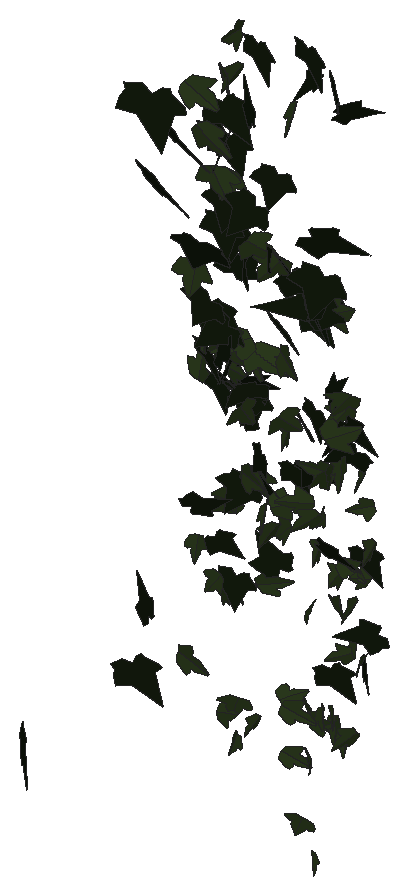
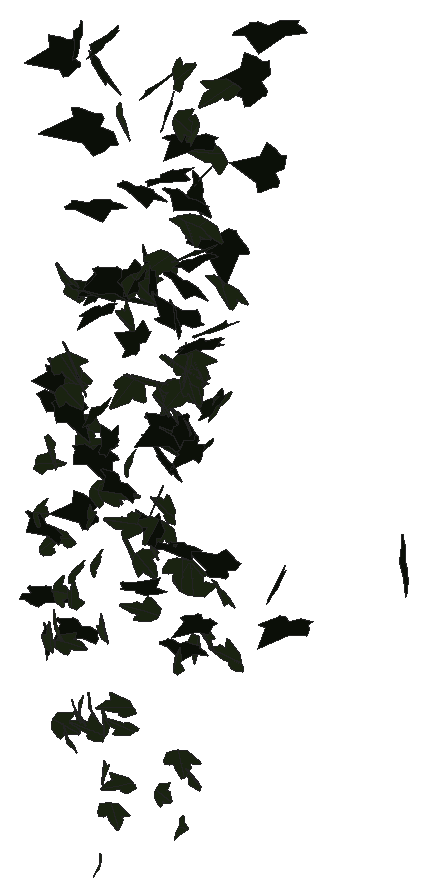
# SketchUp Ruby script. Lengths in inches.
U = 1.inch
M = Sketchup.active_model
def pt(a) = Geom::Point3d.new(a.map { |v| v * U })
def face(e, loops, mat)
  f = e.add_face(loops[0].map { |a| pt(a) })
  loops[1..].each { |l| e.add_face(l.map { |a| pt(a) }).erase! }
  f.material = f.back_material = mat if mat
  f
end
# faces: each face lists its corners as indices into pts; further lists are holes
def faces(e, pts, list, mat = nil) = list.each { |f| face(e, (f[0].is_a?(Array) ? f : [f]).map { |l| l.map { |i| pts[i] } }, mat) }
# xy, xz, yz: faces in a plane at the given z, y or x. An outline is a flat list of corners, or four numbers for a rectangle; further outlines are holes
def ring(l) = l.size == 4 ? [[l[0], l[1]], [l[2], l[1]], [l[2], l[3]], [l[0], l[3]]] : l.each_slice(2).to_a
def flat(e, list, mat, &to3) = list.each { |f| face(e, (f[0].is_a?(Array) ? f : [f]).map { |l| ring(l).map { |u, v| to3.(u, v) } }, mat) }
def xy(e, z, list, mat = nil) = flat(e, list, mat) { |x, y| [x, y, z] }
def xz(e, y, list, mat = nil) = flat(e, list, mat) { |x, z| [x, y, z] }
def yz(e, x, list, mat = nil) = flat(e, list, mat) { |y, z| [x, y, z] }
def lines(e, pts, list) = list.each { |a, b| e.add_line(pt(pts[a]), pt(pts[b])) }
# prism: a flat outline (further loops are holes) pulled along v
def prism(e, loops, v, mat = nil)
  f = face(e, loops, mat); d = Geom::Vector3d.new(v.map { |x| x * U })
  f.pushpull(f.normal.samedirection?(d) ? d.length : -d.length)
end
def box(e, o, s, mat = nil) = prism(e, [[o, [o[0] + s[0], o[1], o[2]], [o[0] + s[0], o[1] + s[1], o[2]], [o[0], o[1] + s[1], o[2]]]], [0, 0, s[2]], mat)
def at(x, y, z, deg = 0) = Geom::Transformation.translation(pt([x, y, z])) * Geom::Transformation.rotation(ORIGIN, Z_AXIS, deg.degrees)
def axes(o, x, y, z) = Geom::Transformation.new([*x, 0, *y, 0, *z, 0, *pt(o).to_a, 1])
def part(name) = M.definitions.add(name)
# library, detail: a bought-in or finely detailed component or shape, given as its bounding box
def library(name, o, s) = part(name).tap { |d| box(d.entities, o, s) }
def detail(e, o, s) = box(e.add_group.entities, o, s)
def put(e, d, t, mat = nil) = e.add_instance(d, t).tap { |i| i.material = mat if mat }
def group(e, t, mat = nil) = e.add_group.tap { |g| g.transformation = t; g.material = mat if mat }.entities
root = M.entities
M.materials.add("1026 AP 7946 SUNNY SIDE UP").color = [254, 231, 186]
M.materials.add("efeu1").color = [18, 25, 13]
M.materials.add("efeu2").color = [43, 57, 29]
c1 = part("ivyleaf_9")
p = [[1.54,2.16,1.25],[1.36,2.04,1.19],[-0.21,0.99,0.68],[-0.71,1.11,0.82],[-0.85,0.86,0.67],[-0.8,0.17,0.21],
  [-0.9,-0.01,0.1],[-0.67,-0.16,-0.02],[-0.08,-0.08,-0.05],[-0.03,-0.6,-0.4],[0.65,-0.88,-0.66],[0.83,-0.6,-0.49],
  [1.29,-0.42,-0.43],[1.8125,-0.07,-0.26],[1.21,0.44,0.15]]
faces(c1.entities,p,[[0,1,2,3,4,5,6,7,8,9,10,11,12,13,14]],"efeu1")
c2 = part("ivyleaf_10")
p = [[0,0.5,-0.03],[-0.0625,2.02,-0.43],[-0.19,2.01,-0.46],[-0.54,1.05,-0.29],[-0.52,0.625,-0.18],[-0.83,0.76,-0.28],
  [-1.16,0.64,-0.33],[-1.15,0.33,-0.24],[-0.77,-0.39,0.02],[-0.3,-0.51,0.16],[0.04,-0.48,0.23],[-0.02,2.01,-0.4375],
  [-0.06,2.01,-0.43],[0.04,-0.49,0.23],[0.67,-0.49,0.14],[1.38,0.36,-0.2],[1.375,0.51,-0.24],[0.81,0.65,-0.19],
  [0.62,0.59,-0.15],[0.6,1.09,-0.28],[0.5,1.23,-0.31]]
faces(c2.entities,p,[[0,1,2,3,4,5,6,7,8,9,10],[11,12,0,13,14,15,16,17,18,19,20]],"efeu2")
put(root,c1,axes([100.33,204.32,252.68],[-0.06689,-0.01486,-0.42781],[0.60698,-0.18066,-0.03309],[-0.3032,-0.35839,0.02813]),"1026 AP 7946 SUNNY SIDE UP")
put(root,c1,axes([100.42,208.17,252.85],[-0.02192,-0.21369,-0.24317],[0.05849,0.22216,-0.22556],[0.52269,-0.03382,0.01504]),"1026 AP 7946 SUNNY SIDE UP")
put(root,c1,axes([100.73,208.45,267.375],[-0.21332,-0.34879,-0.14264],[0.07351,0.12119,-0.39521],[0.6268,-0.13292,-0.00219]),"1026 AP 7946 SUNNY SIDE UP")
put(root,c1,axes([100.34,208.77,253.88],[-0.06453,-0.21774,0.20723],[0.12356,0.18485,0.23705],[-0.4822,0.0765,0.03301]),"1026 AP 7946 SUNNY SIDE UP")
put(root,c1,axes([100.54,209.02,266.34],[0.46908,-0.21894,0.12393],[0.1304,-0.0936,-0.37784],[0.40208,0.28577,-0.02204]),"1026 AP 7946 SUNNY SIDE UP")
put(root,c1,axes([99.8125,209.43,264.58],[0.34989,-0.20333,0.18498],[0.18034,-0.14138,-0.31102],[0.41869,0.23081,-0.02062]),"1026 AP 7946 SUNNY SIDE UP")
put(root,c2,axes([100.67,209.64,252.51],[0.05499,0.01025,0.28287],[0.44485,-0.03571,-0.03343],[0.05811,0.26366,-0.01177]),"1026 AP 7946 SUNNY SIDE UP")
put(root,c1,axes([100.82,209.99,262.9375],[0.38336,0.11623,-0.22338],[-0.31768,-0.09566,-0.27325],[-0.25553,0.29329,0.00457]),"1026 AP 7946 SUNNY SIDE UP")
put(root,c1,axes([104.2,209.9,264.33],[0.06546,0.07746,-0.3305],[0.2079,0.29284,0.09211],[0.47621,-0.1385,0.00522]),"1026 AP 7946 SUNNY SIDE UP")
put(root,c1,axes([102.03,210.44,264.12],[-0.25853,-0.23144,0.13813],[-0.09867,-0.12119,-0.29264],[0.40991,-0.17515,0.01667]),"1026 AP 7946 SUNNY SIDE UP")
put(root,c2,axes([100.36,210.37,262.02],[0.49444,-0.07924,0.04839],[0.064,-0.03693,-0.32253],[0.14199,0.2926,-0.02315]),"1026 AP 7946 SUNNY SIDE UP")
put(root,c2,axes([100.48,210.18,266.73],[0.1459,0.22857,0.21376],[0.15113,0.17617,-0.25837],[-0.48907,0.12262,-0.01607]),"1026 AP 7946 SUNNY SIDE UP")
put(root,c2,axes([101.85,210.25,258.98],[-0.1197,-0.24997,-0.17319],[0.11301,0.15182,-0.26746],[0.45872,-0.10263,0.02069]),"1026 AP 7946 SUNNY SIDE UP")
put(root,c1,axes([103.89,210.57,262.89],[-0.31774,-0.25711,-0.03842],[0.05746,0.01679,-0.33627],[0.40413,-0.20454,0.0176]),"1026 AP 7946 SUNNY SIDE UP")
put(root,c1,axes([100.5,210.75,261.03],[-0.22644,-0.20621,0.16767],[0.00213,-0.17947,-0.25009],[0.44234,-0.1047,0.08704]),"1026 AP 7946 SUNNY SIDE UP")
put(root,c2,axes([102.66,210.67,260.39],[0.08325,-0.0002,0.31918],[0.42935,-0.14849,-0.04904],[0.23019,0.27703,-0.02397]),"1026 AP 7946 SUNNY SIDE UP")
put(root,c1,axes([100.96,210.8,260.53],[-0.28596,-0.17425,0.17453],[-0.128,-0.15333,-0.25744],[0.3871,-0.17942,0.04381]),"1026 AP 7946 SUNNY SIDE UP")
put(root,c2,axes([100.43,210.67,265.38],[-0.26576,0.01315,-0.26616],[0.3743,-0.12946,-0.15768],[-0.19685,-0.2639,0.05951]),"1026 AP 7946 SUNNY SIDE UP")
put(root,c2,axes([100.17,210.73,254.82],[0.31007,-0.10493,0.10073],[0.11794,-0.0695,-0.2251],[0.20994,0.19402,-0.02231]),"1026 AP 7946 SUNNY SIDE UP")
put(root,c1,axes([101.14,210.46,259.92],[-0.02232,0.09727,0.29593],[-0.05622,0.28447,-0.09959],[-0.47272,-0.03842,-0.00213]),"1026 AP 7946 SUNNY SIDE UP")
put(root,c2,axes([102.74,210.59,258.9],[-0.16914,-0.1943,-0.22602],[0.17819,0.18668,-0.22761],[0.42356,-0.15612,0.0055]),"1026 AP 7946 SUNNY SIDE UP")
put(root,c2,axes([100.33,210.59,259.23],[0.06679,0.20154,-0.21646],[0.0174,0.21222,0.21211],[0.45878,-0.03739,0.02347]),"1026 AP 7946 SUNNY SIDE UP")
put(root,c2,axes([100.9,210.94,260.3],[-0.28728,-0.19996,0.11794],[-0.08575,-0.10423,-0.28047],[0.38015,-0.17462,0.02586]),"1026 AP 7946 SUNNY SIDE UP")
put(root,c2,axes([103.05,210.88,248.6],[-0.30964,-0.02592,0.07216],[-0.10313,-0.03532,-0.2032],[0.05663,-0.20605,0.02449]),"1026 AP 7946 SUNNY SIDE UP")
put(root,c1,axes([100.57,210.84,260.79],[0.10046,-0.21763,-0.19662],[0.02676,0.18698,-0.23279],[0.47957,0.03515,0.05418]),"1026 AP 7946 SUNNY SIDE UP")
put(root,c2,axes([103.74,210.84,257.73],[-0.06962,-0.26214,-0.10878],[0.04478,0.10068,-0.27308],[0.44124,-0.05158,0.01055]),"1026 AP 7946 SUNNY SIDE UP")
put(root,c1,axes([103.9,210.89,252.74],[-0.10489,-0.11251,-0.22048],[0.22622,0.15915,-0.13185],[0.30446,-0.15701,0.02201]),"1026 AP 7946 SUNNY SIDE UP")
put(root,c2,axes([103.24,211.06,256.34],[-0.09031,-0.13936,0.20787],[-0.10508,-0.19135,-0.15625],[0.37207,-0.08787,0.00633]),"1026 AP 7946 SUNNY SIDE UP")
put(root,c2,axes([103.93,210.875,258.71],[0.28807,-0.02878,-0.22722],[0.34943,0.02915,0.18655],[0.00665,-0.28511,0.0403]),"1026 AP 7946 SUNNY SIDE UP")
put(root,c2,axes([100.56,210.94,253.91],[0.27863,-0.14001,-0.06444],[-0.08614,0.03036,-0.23032],[0.24266,0.17154,-0.00777]),"1026 AP 7946 SUNNY SIDE UP")
put(root,c2,axes([103.97,211.08,257.96],[0.29834,-0.16178,0.17139],[0.19249,-0.11417,-0.25746],[0.3112,0.22572,-0.00505]),"1026 AP 7946 SUNNY SIDE UP")
put(root,c2,axes([101.26,211.04,260.16],[-0.34906,0.18703,0.13524],[-0.38078,-0.16887,-0.12801],[-0.00575,-0.17062,0.26737]),"1026 AP 7946 SUNNY SIDE UP")
put(root,c1,axes([99.95,210.9,255.53],[0.0332,-0.00464,0.23861],[0.37779,0.01438,-0.02038],[-0.02364,0.22333,0.00941]),"1026 AP 7946 SUNNY SIDE UP")
put(root,c1,axes([100.08,211.12,259.52],[0.13049,-0.22686,0.10431],[0.04348,-0.09729,-0.2577],[0.41888,0.08077,-0.00575]),"1026 AP 7946 SUNNY SIDE UP")
put(root,c1,axes([100.6,211.14,262.93],[-0.09336,-0.26313,-0.026],[0.01497,0.01946,-0.28747],[0.44782,-0.05551,0.00419]),"1026 AP 7946 SUNNY SIDE UP")
put(root,c2,axes([100.75,211.09,259.94],[-0.06878,-0.29267,0.05362],[-0.00736,-0.05361,-0.30515],[0.46782,-0.04387,0.00308]),"1026 AP 7946 SUNNY SIDE UP")
put(root,c2,axes([102.61,210.95,251.26],[0.1064,0.06801,0.22713],[0.29392,0.11784,-0.09604],[-0.21168,0.19781,-0.01918]),"1026 AP 7946 SUNNY SIDE UP")
put(root,c1,axes([103.53,211.02,255.71],[0.34424,-0.06958,0.1098],[0.1497,-0.05241,-0.23614],[0.13362,0.23796,-0.01833]),"1026 AP 7946 SUNNY SIDE UP")
put(root,c1,axes([101.53,210.95,265.97],[-0.06073,-0.14612,0.27545],[0.07527,0.26411,0.15688],[-0.47432,0.06062,-0.01038]),"1026 AP 7946 SUNNY SIDE UP")
put(root,c2,axes([100.89,210.94,260.27],[0.14703,-0.19167,-0.2129],[0.03563,0.20994,-0.20654],[0.46445,0.04457,0.08324]),"1026 AP 7946 SUNNY SIDE UP")
put(root,c2,axes([102.87,211.23,256.51],[-0.02273,0.01089,0.25684],[-0.23833,-0.1987,-0.00128],[0.31161,-0.15118,0.01776]),"1026 AP 7946 SUNNY SIDE UP")
put(root,c2,axes([100.64,211.04,253.6],[-0.23749,0.15188,0.08361],[-0.10917,0.04392,-0.21975],[-0.26693,-0.15309,0.01549]),"1026 AP 7946 SUNNY SIDE UP")
put(root,c2,axes([101.17,211.23,256.59],[-0.02039,0.02083,0.27185],[0.39699,-0.07801,0.01868],[0.12442,0.2523,-0.01504]),"1026 AP 7946 SUNNY SIDE UP")
put(root,c1,axes([104.32,211.18,258.34],[0.07273,0.04407,-0.25909],[-0.30511,-0.16045,-0.0666],[-0.26155,0.19943,0.00564]),"1026 AP 7946 SUNNY SIDE UP")
put(root,c2,axes([100.48,211.25,250.3125],[0.08272,-0.10399,-0.19767],[0.23887,-0.12344,0.11145],[-0.24525,-0.15531,0.04188]),"1026 AP 7946 SUNNY SIDE UP")
put(root,c2,axes([103.46,211.26,257.46],[-0.10364,-0.00957,-0.25238],[-0.37377,-0.05939,0.06795],[-0.09404,0.24659,0.00809]),"1026 AP 7946 SUNNY SIDE UP")
put(root,c1,axes([100.44,211.34,264.87],[0.04934,-0.26759,-0.03924],[0.07232,-0.02838,0.28473],[-0.45198,-0.03375,0.04127]),"1026 AP 7946 SUNNY SIDE UP")
put(root,c1,axes([100.59,211.18,265.92],[-0.05152,-0.22182,-0.23308],[0.11418,0.21485,-0.22786],[0.4835,-0.07437,0.02898]),"1026 AP 7946 SUNNY SIDE UP")
put(root,c1,axes([103.01,211.36,261.42],[0.13762,-0.24208,0.14419],[0.05291,-0.13792,-0.26563],[0.43758,0.09281,-0.01323]),"1026 AP 7946 SUNNY SIDE UP")
put(root,c2,axes([100.9375,211.23,250.77],[-0.29742,-0.11953,0.04343],[-0.04078,-0.03887,-0.22993],[0.19544,-0.19,0.01812]),"1026 AP 7946 SUNNY SIDE UP")
put(root,c1,axes([100.51,211.01,264.45],[0.05667,0.0287,0.29676],[0.13406,0.26637,-0.03604],[-0.45301,0.08242,0.02646]),"1026 AP 7946 SUNNY SIDE UP")
put(root,c2,axes([100.26,211.3,263.99],[-0.4389,-0.04715,-0.12335],[0.21033,-0.10304,-0.25531],[-0.00372,-0.26337,0.11762]),"1026 AP 7946 SUNNY SIDE UP")
put(root,c1,axes([101.23,211.46,258.83],[-0.42968,-0.09124,-0.06742],[0.17998,-0.15948,-0.2151],[0.05097,-0.20604,0.19118]),"1026 AP 7946 SUNNY SIDE UP")
put(root,c2,axes([101.54,211.42,255.82],[0.17047,-0.11044,0.22753],[0.21452,-0.17508,-0.15976],[0.32469,0.17366,-0.0139]),"1026 AP 7946 SUNNY SIDE UP")
put(root,c2,axes([103.02,211.33,247.49],[-0.0511,0.15842,-0.1256],[0.03287,-0.12106,-0.16728],[-0.31347,-0.03852,0.00293]),"1026 AP 7946 SUNNY SIDE UP")
put(root,c2,axes([103.17,211.39,251.22],[0.14238,-0.06252,0.19355],[0.21846,-0.12769,-0.11328],[0.22258,0.16531,-0.01262]),"1026 AP 7946 SUNNY SIDE UP")
put(root,c2,axes([100.84,211.21,259.74],[-0.29307,-0.16204,-0.15047],[0.20867,0.06983,-0.25065],[0.29555,-0.20999,0.02776]),"1026 AP 7946 SUNNY SIDE UP")
put(root,c1,axes([103.48,211.44,267.38],[0.07404,-0.04087,-0.28433],[0.38262,-0.13044,0.06196],[-0.21389,-0.24748,0.01241]),"1026 AP 7946 SUNNY SIDE UP")
put(root,c1,axes([100.4,211.49,263.25],[-0.13377,-0.24507,0.10587],[0.04543,-0.11328,-0.27059],[0.44836,-0.06164,0.05901]),"1026 AP 7946 SUNNY SIDE UP")
put(root,c2,axes([101.4,211.17,262.65],[-0.17261,-0.17685,-0.2413],[0.26972,0.16296,-0.20952],[0.37291,-0.19972,0.03985]),"1026 AP 7946 SUNNY SIDE UP")
put(root,c2,axes([101.36,211.38,259.74],[-0.19248,-0.20878,-0.20912],[0.47848,-0.10842,-0.05333],[-0.05982,-0.19545,0.24629]),"1026 AP 7946 SUNNY SIDE UP")
put(root,c1,axes([103.18,211.3125,257.4375],[0.1615,0.12928,-0.19414],[-0.1741,-0.1535,-0.17089],[-0.31544,0.15092,-0.00507]),"1026 AP 7946 SUNNY SIDE UP")
put(root,c1,axes([104,211.36,258.83],[0.00905,-0.03052,-0.26257],[0.38765,0.07107,-0.00262],[0.11148,-0.24465,0.03042]),"1026 AP 7946 SUNNY SIDE UP")
put(root,c1,axes([103.18,211.56,261.57],[0.09415,-0.13697,-0.24899],[0.21051,-0.20151,0.15112],[-0.38153,-0.14498,0.02194]),"1026 AP 7946 SUNNY SIDE UP")
put(root,c1,axes([103.32,211.5,261.49],[-0.64265,0.1358,0.11479],[-0.28064,-0.21746,-0.33862],[-0.08017,-0.32734,0.26521]),"1026 AP 7946 SUNNY SIDE UP")
put(root,c1,axes([100.18,211.48,258.53],[0.04007,-0.2284,0.0783],[0.02278,-0.07511,-0.2468],[0.40804,0.02662,0.00609]),"1026 AP 7946 SUNNY SIDE UP")
put(root,c2,axes([101.77,211.47,255.38],[-0.05167,-0.2221,0.13415],[-0.02091,-0.1309,-0.232],[0.4053,-0.03507,0.00513]),"1026 AP 7946 SUNNY SIDE UP")
put(root,c2,axes([100.55,211.49,259.01],[0.0517,-0.05727,-0.24847],[0.24851,-0.17954,0.06571],[-0.31925,-0.14903,0.01092]),"1026 AP 7946 SUNNY SIDE UP")
put(root,c2,axes([101.7,211.25,254],[-0.0861,-0.04802,0.2345],[0.21173,0.18449,0.07446],[-0.2988,0.14457,-0.01481]),"1026 AP 7946 SUNNY SIDE UP")
put(root,c2,axes([103.89,211.44,259.44],[-0.2424,-0.16604,0.12146],[-0.10798,-0.09807,-0.2335],[0.30236,-0.16813,0.01398]),"1026 AP 7946 SUNNY SIDE UP")
put(root,c1,axes([102,211.35,254.51],[-0.3597,-0.12383,0.02501],[0.02633,0.02149,0.26787],[-0.19688,0.22912,-0.00987]),"1026 AP 7946 SUNNY SIDE UP")
put(root,c1,axes([101.8125,211.52,260.63],[0.16934,-0.21477,0.15497],[0.11207,-0.13389,-0.24827],[0.39792,0.12911,0.00397]),"1026 AP 7946 SUNNY SIDE UP")
put(root,c1,axes([101.12,211.58,258.41],[-0.33934,-0.15421,-0.07827],[0.25312,-0.10686,-0.20219],[0.13792,-0.18329,0.17849]),"1026 AP 7946 SUNNY SIDE UP")
put(root,c1,axes([101.87,211.49,264.38],[-0.34006,-0.12005,-0.10618],[0.1568,0.03062,-0.25381],[0.19226,-0.23731,0.0192]),"1026 AP 7946 SUNNY SIDE UP")
put(root,c2,axes([103.48,211.49,251.04],[0.2521,-0.1197,0.13092],[0.14853,-0.08672,-0.20632],[0.23178,0.18576,-0.01018]),"1026 AP 7946 SUNNY SIDE UP")
put(root,c2,axes([102.75,211.52,249.75],[-0.09804,0.04162,0.21158],[0.20353,-0.16055,0.07315],[0.25866,0.1421,0.02264]),"1026 AP 7946 SUNNY SIDE UP")
put(root,c1,axes([101.44,211.54,262.15],[-0.04672,0.06487,0.28408],[0.05095,-0.2743,0.06856],[0.44194,0.03848,0.02213]),"1026 AP 7946 SUNNY SIDE UP")
put(root,c2,axes([103.37,211.55,251.14],[0.00244,-0.0391,0.22842],[0.23332,-0.16688,-0.03233],[0.26672,0.14634,0.02619]),"1026 AP 7946 SUNNY SIDE UP")
put(root,c2,axes([100.48,211.46,263.93],[0.44537,-0.03153,0.00958],[0.01043,-0.02696,-0.2819],[0.05485,0.26114,-0.02421]),"1026 AP 7946 SUNNY SIDE UP")
put(root,c2,axes([101.11,211.55,259.42],[0.13287,-0.01504,0.27096],[0.347,-0.14699,-0.08253],[0.2265,0.23401,-0.03252]),"1026 AP 7946 SUNNY SIDE UP")
put(root,c2,axes([104.42,211.55,256.8125],[0.05773,0.01466,-0.21602],[-0.22945,-0.15155,-0.03811],[-0.23808,0.14961,-0.01566]),"1026 AP 7946 SUNNY SIDE UP")
put(root,c1,axes([104.61,211.57,253.6],[-0.05683,-0.09706,-0.22992],[-0.15207,-0.20072,0.10514],[-0.35031,0.10288,-0.00834]),"1026 AP 7946 SUNNY SIDE UP")
put(root,c2,axes([100.63,211.66,267.58],[-0.0115,-0.00843,-0.30621],[-0.10019,-0.29033,0.0084],[-0.45663,0.06391,0.00586]),"1026 AP 7946 SUNNY SIDE UP")
put(root,c1,axes([100.66,211.52,253.72],[-0.25432,-0.15908,-0.11002],[0.14158,0.05893,-0.23253],[0.26505,-0.18412,0.01864]),"1026 AP 7946 SUNNY SIDE UP")
put(root,c2,axes([101.83,211.55,262.14],[-0.24364,-0.17386,0.1723],[-0.11991,-0.15451,-0.23774],[0.36103,-0.16865,0.03732]),"1026 AP 7946 SUNNY SIDE UP")
put(root,c2,axes([102.19,211.41,255.5625],[0.1871,-0.19896,-0.13043],[-0.12221,0.09946,-0.23782],[0.34909,0.14145,-0.01335]),"1026 AP 7946 SUNNY SIDE UP")
put(root,c1,axes([103.76,211.47,258.45],[-0.08353,0.22862,-0.14995],[0.04305,-0.14436,-0.24259],[-0.42509,-0.05955,0.0049]),"1026 AP 7946 SUNNY SIDE UP")
put(root,c1,axes([102.31,211.52,257.09],[-0.14251,-0.05147,-0.2274],[0.33232,0.06585,-0.10497],[0.12755,-0.22907,0.01941]),"1026 AP 7946 SUNNY SIDE UP")
put(root,c2,axes([103.84,211.44,255.15],[0.16333,0.06582,0.17563],[0.25427,0.05734,-0.12424],[-0.13269,0.19089,-0.02189]),"1026 AP 7946 SUNNY SIDE UP")
put(root,c1,axes([103.875,211.27,266.78],[0.21756,0.11278,0.22866],[0.29125,0.12195,-0.18261],[-0.26024,0.23077,-0.01321]),"1026 AP 7946 SUNNY SIDE UP")
put(root,c1,axes([100.57,211.57,262.61],[-0.32103,-0.06944,-0.16619],[0.26664,0.01411,-0.21266],[0.10693,-0.24368,0.03135]),"1026 AP 7946 SUNNY SIDE UP")
put(root,c2,axes([103.86,211.63,250.74],[-0.05428,-0.14534,0.19691],[-0.05441,-0.18892,-0.15487],[0.37467,-0.04849,0.00604]),"1026 AP 7946 SUNNY SIDE UP")
put(root,c1,axes([101.23,211.6875,256.96],[0.12086,-0.12968,-0.2323],[0.26649,-0.15241,0.14942],[-0.30896,-0.18219,0.03801]),"1026 AP 7946 SUNNY SIDE UP")
put(root,c1,axes([100.85,211.63,256.11],[-0.3376,-0.15769,-0.00509],[0.02434,-0.01425,-0.27369],[0.24684,-0.21427,0.02002]),"1026 AP 7946 SUNNY SIDE UP")
put(root,c1,axes([101.8,211.6,262.17],[0.22397,-0.16282,0.14837],[0.1327,-0.11846,-0.22321],[0.31604,0.16513,-0.01142]),"1026 AP 7946 SUNNY SIDE UP")
put(root,c1,axes([100.95,211.5,257.84],[-0.11584,0.16815,0.19568],[0.13886,-0.16736,0.18789],[0.37274,0.11461,-0.00918]),"1026 AP 7946 SUNNY SIDE UP")
put(root,c2,axes([102.65,211.59,250.94],[-0.15671,0.10703,0.15709],[0.18737,-0.09542,0.14927],[0.22416,0.15458,-0.01494]),"1026 AP 7946 SUNNY SIDE UP")
put(root,c1,axes([102.81,211.69,258.6],[0.03598,-0.23331,0.13741],[0.02031,-0.13409,-0.24229],[0.42313,0.02627,-0.00005]),"1026 AP 7946 SUNNY SIDE UP")
put(root,c2,axes([102,211.35,256.09],[0.09711,0.02781,-0.28285],[0.32191,0.18428,0.06771],[0.29133,-0.21289,0.01946]),"1026 AP 7946 SUNNY SIDE UP")
put(root,c2,axes([100.25,211.56,266.46],[-0.18905,0.22487,-0.11519],[0.07766,-0.10067,-0.27002],[-0.41819,-0.12035,0.00193]),"1026 AP 7946 SUNNY SIDE UP")
put(root,c2,axes([104.23,211.66,254.86],[-0.02994,0.09151,0.20283],[0.01493,-0.19658,0.09417],[0.34032,0.01667,0.01372]),"1026 AP 7946 SUNNY SIDE UP")
put(root,c2,axes([102.21,211.44,249.75],[0.10522,0.08931,0.19275],[0.2139,0.12875,-0.11299],[-0.24505,0.15073,-0.01586]),"1026 AP 7946 SUNNY SIDE UP")
put(root,c2,axes([104.375,211.71,255.69],[-0.01305,-0.11034,0.22353],[0.12636,-0.20682,-0.10609],[0.36223,0.06817,0.04506]),"1026 AP 7946 SUNNY SIDE UP")
put(root,c2,axes([103.73,211.66,252.76],[-0.07014,-0.04962,0.20038],[-0.14068,-0.17377,-0.06772],[0.28303,-0.09867,0.01599]),"1026 AP 7946 SUNNY SIDE UP")
put(root,c2,axes([103.39,211.625,261.36],[0.21763,-0.1265,-0.23407],[0.28728,-0.13471,0.19175],[-0.28959,-0.22871,0.01431]),"1026 AP 7946 SUNNY SIDE UP")
put(root,c2,axes([102.91,211.54,250.81],[0.00261,-0.00243,0.24046],[0.36101,0.04224,-0.00098],[-0.06639,0.22958,0.00411]),"1026 AP 7946 SUNNY SIDE UP")
put(root,c1,axes([104.17,211.68,252.66],[-0.01404,-0.02455,-0.25419],[0.35915,-0.09656,0.00082],[-0.15119,-0.22709,0.02555]),"1026 AP 7946 SUNNY SIDE UP")
put(root,c2,axes([100.53,211.71,266.55],[0.02443,-0.20752,0.19753],[0.03897,-0.18595,-0.22515],[0.47284,0.02604,0.00835]),"1026 AP 7946 SUNNY SIDE UP")
put(root,c1,axes([102.58,211.71,267.74],[0.10912,-0.28999,0.08224],[0.02154,-0.08049,-0.3076],[0.47314,0.07054,-0.00496]),"1026 AP 7946 SUNNY SIDE UP")
put(root,c1,axes([100.28,211.5,258.7],[0.38036,-0.06279,-0.0838],[-0.12332,0.0277,-0.24863],[0.11594,0.23545,0.01046]),"1026 AP 7946 SUNNY SIDE UP")
put(root,c2,axes([102.99,211.71,256.05],[-0.01535,0.05205,-0.20364],[-0.00338,-0.19821,-0.05474],[-0.32185,-0.0004,0.01029]),"1026 AP 7946 SUNNY SIDE UP")
put(root,c1,axes([100.64,211.51,261.54],[-0.19267,0.00456,0.23927],[0.37877,-0.0118,0.12144],[0.02137,0.25033,0.00488]),"1026 AP 7946 SUNNY SIDE UP")
put(root,c1,axes([101.19,211.72,256.25],[0.08591,-0.08998,0.23962],[0.14717,-0.21387,-0.1089],[0.36429,0.10762,-0.01251]),"1026 AP 7946 SUNNY SIDE UP")
put(root,c1,axes([102.37,211.45,261.99],[-0.01817,-0.04273,-0.29618],[0.14042,0.27304,-0.04394],[0.43453,-0.09002,0.00181]),"1026 AP 7946 SUNNY SIDE UP")
put(root,c1,axes([100.64,211.71,261.75],[-0.04669,-0.03751,-0.25681],[0.39156,-0.07784,-0.0164],[-0.12597,-0.22804,0.0442]),"1026 AP 7946 SUNNY SIDE UP")
put(root,c2,axes([103.625,211.7,258.91],[-0.17665,-0.16996,0.15586],[-0.05041,-0.15627,-0.20499],[0.35524,-0.10669,0.04842]),"1026 AP 7946 SUNNY SIDE UP")
put(root,c1,axes([100.36,211.66,264.73],[-0.22292,-0.12553,-0.20451],[0.31342,0.06854,-0.18473],[0.2248,-0.22003,0.05476]),"1026 AP 7946 SUNNY SIDE UP")
put(root,c2,axes([104.0625,211.7,252.57],[0.03547,-0.17947,-0.1403],[0.031,-0.13374,0.18555],[-0.35192,-0.02987,0.0022]),"1026 AP 7946 SUNNY SIDE UP")
put(root,c1,axes([103.26,211.63,259.16],[-0.03179,0.19191,0.23209],[0.03875,-0.22284,0.19749],[0.46242,0.03187,-0.00059]),"1026 AP 7946 SUNNY SIDE UP")
put(root,c1,axes([102.8,211.57,261.15],[0.06264,-0.20722,-0.15754],[-0.01358,0.15239,-0.21583],[0.40363,0.03728,0.01719]),"1026 AP 7946 SUNNY SIDE UP")
put(root,c2,axes([103.8,211.77,254],[0.07153,-0.10925,0.22608],[0.10283,-0.21036,-0.12274],[0.37241,0.07907,-0.00953]),"1026 AP 7946 SUNNY SIDE UP")
put(root,c2,axes([102.07,211.51,251.14],[0.19355,-0.01094,-0.1774],[0.2553,0.07872,0.11491],[0.09154,-0.19643,0.05459]),"1026 AP 7946 SUNNY SIDE UP")
put(root,c2,axes([101.91,211.76,257.75],[-0.03051,-0.08661,0.22707],[0.18076,-0.19732,-0.07045],[0.32638,0.10119,0.06024]),"1026 AP 7946 SUNNY SIDE UP")
put(root,c2,axes([102.1,211.75,266.08],[0.24479,-0.20095,0.16773],[0.13269,-0.14157,-0.26213],[0.38562,0.17628,-0.01628]),"1026 AP 7946 SUNNY SIDE UP")
put(root,c2,axes([103.35,211.79,254.61],[-0.10526,-0.03223,0.23409],[0.12903,-0.2246,-0.00922],[0.33732,0.07585,0.07657]),"1026 AP 7946 SUNNY SIDE UP")
put(root,c2,axes([100.7,211.61,253.1875],[-0.21531,0.14737,0.02465],[0.03663,-0.00924,0.20774],[0.25005,0.12825,-0.0092]),"1026 AP 7946 SUNNY SIDE UP")
put(root,c2,axes([100.23,211.64,255.28],[-0.34942,-0.13481,0.0042],[-0.00814,0.01785,0.26723],[-0.21196,0.22156,-0.01719]),"1026 AP 7946 SUNNY SIDE UP")
put(root,c1,axes([100.52,211.74,259.18],[-0.11273,0.05684,-0.23254],[0.19645,-0.18633,-0.09238],[-0.32803,-0.13113,0.02459]),"1026 AP 7946 SUNNY SIDE UP")
put(root,c2,axes([103.48,211.65,253.81],[-0.27635,0.12595,0.05587],[0.08183,-0.01905,0.22214],[0.19902,0.18273,-0.01377]),"1026 AP 7946 SUNNY SIDE UP")
put(root,c1,axes([100.1,211.54,254.5],[0.0163,-0.07466,-0.21835],[0.02728,0.20286,-0.07624],[0.36612,-0.01179,0.0154]),"1026 AP 7946 SUNNY SIDE UP")
put(root,c2,axes([101.03,211.76,250.09],[0.00634,-0.14995,0.15031],[0.03142,-0.14584,-0.15493],[0.32841,0.01685,0.01192]),"1026 AP 7946 SUNNY SIDE UP")
put(root,c1,axes([100.93,211.46,258.79],[0.28549,0.13895,0.1524],[0.18964,0.08539,-0.23231],[-0.27675,0.20185,-0.00197]),"1026 AP 7946 SUNNY SIDE UP")
put(root,c2,axes([101.125,211.62,256.44],[-0.38841,-0.00832,-0.10943],[0.16746,-0.02076,-0.2537],[-0.00091,-0.26807,0.02147]),"1026 AP 7946 SUNNY SIDE UP")
put(root,c2,axes([104.14,211.64,257.4375],[0.13461,-0.23151,-0.05523],[-0.03417,0.04772,-0.25397],[0.37163,0.08824,-0.00335]),"1026 AP 7946 SUNNY SIDE UP")
put(root,c2,axes([100.49,211.76,249.4375],[0.00312,0.11733,-0.17708],[-0.03294,-0.17158,-0.12144],[-0.32645,0.01843,0.01056]),"1026 AP 7946 SUNNY SIDE UP")
put(root,c2,axes([102.76,211.82,255.05],[-0.03139,-0.08153,0.22931],[0.17258,-0.20166,-0.067],[0.33114,0.09737,0.05665]),"1026 AP 7946 SUNNY SIDE UP")
put(root,c1,axes([104.17,211.71,255.49],[-0.13755,-0.07086,-0.23461],[0.34508,0.06999,-0.10906],[0.14529,-0.23331,0.03692]),"1026 AP 7946 SUNNY SIDE UP")
put(root,c2,axes([100.51,211.66,255.75],[-0.33116,-0.1578,-0.00502],[0.02409,-0.01383,-0.27039],[0.24703,-0.21019,0.01963]),"1026 AP 7946 SUNNY SIDE UP")
put(root,c1,axes([102.83,211.71,267.2],[-0.33018,0.13296,-0.12784],[0.14924,-0.08293,-0.25591],[-0.2449,-0.22979,0.01641]),"1026 AP 7946 SUNNY SIDE UP")
put(root,c1,axes([101.05,211.81,267.28],[0.06645,-0.27663,0.05016],[0.00221,-0.05076,-0.29975],[0.47733,0.03875,-0.0056]),"1026 AP 7946 SUNNY SIDE UP")
put(root,c2,axes([102.52,211.78,253.375],[0.04109,-0.15953,-0.14943],[0.07227,-0.1377,0.16478],[-0.33025,-0.04999,0.01747]),"1026 AP 7946 SUNNY SIDE UP")
put(root,c2,axes([103.8,211.81,253.15],[0.13107,-0.059,0.23081],[0.23526,-0.16855,-0.1039],[0.27882,0.16995,-0.02083]),"1026 AP 7946 SUNNY SIDE UP")
put(root,c1,axes([102.33,211.84,258.09],[0.04262,-0.13079,0.21249],[0.07427,-0.20157,-0.13875],[0.3778,0.05438,0.0033]),"1026 AP 7946 SUNNY SIDE UP")
put(root,c2,axes([103.51,211.77,250.54],[0.21223,-0.08676,0.15473],[0.17416,-0.10415,-0.16459],[0.21076,0.17343,-0.0198]),"1026 AP 7946 SUNNY SIDE UP")
